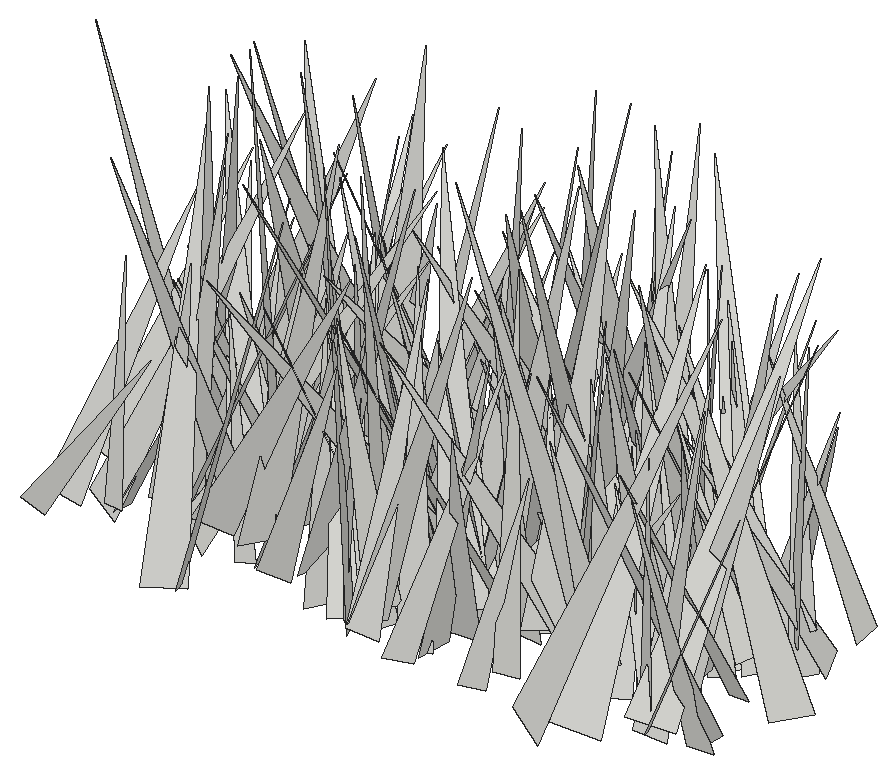
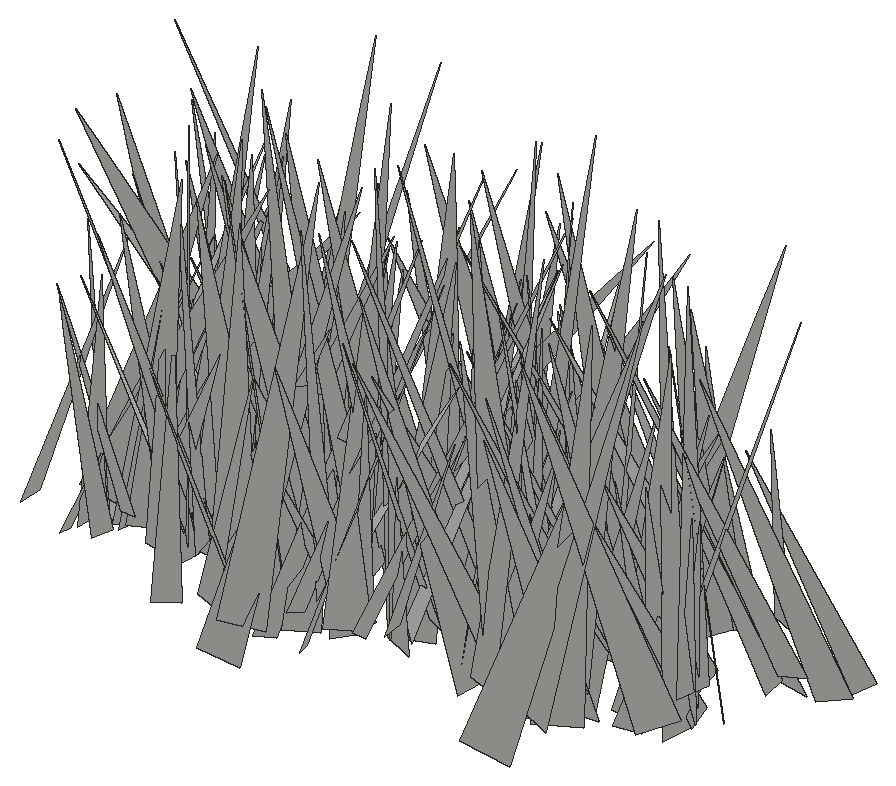
# SketchUp Ruby script. Lengths in inches.
U = 1.inch
M = Sketchup.active_model
def pt(a) = Geom::Point3d.new(a.map { |v| v * U })
def face(e, loops, mat)
  f = e.add_face(loops[0].map { |a| pt(a) })
  loops[1..].each { |l| e.add_face(l.map { |a| pt(a) }).erase! }
  f.material = f.back_material = mat if mat
  f
end
# faces: each face lists its corners as indices into pts; further lists are holes
def faces(e, pts, list, mat = nil) = list.each { |f| face(e, (f[0].is_a?(Array) ? f : [f]).map { |l| l.map { |i| pts[i] } }, mat) }
# xy, xz, yz: faces in a plane at the given z, y or x. An outline is a flat list of corners, or four numbers for a rectangle; further outlines are holes
def ring(l) = l.size == 4 ? [[l[0], l[1]], [l[2], l[1]], [l[2], l[3]], [l[0], l[3]]] : l.each_slice(2).to_a
def flat(e, list, mat, &to3) = list.each { |f| face(e, (f[0].is_a?(Array) ? f : [f]).map { |l| ring(l).map { |u, v| to3.(u, v) } }, mat) }
def xy(e, z, list, mat = nil) = flat(e, list, mat) { |x, y| [x, y, z] }
def xz(e, y, list, mat = nil) = flat(e, list, mat) { |x, z| [x, y, z] }
def yz(e, x, list, mat = nil) = flat(e, list, mat) { |y, z| [x, y, z] }
def lines(e, pts, list) = list.each { |a, b| e.add_line(pt(pts[a]), pt(pts[b])) }
# prism: a flat outline (further loops are holes) pulled along v
def prism(e, loops, v, mat = nil)
  f = face(e, loops, mat); d = Geom::Vector3d.new(v.map { |x| x * U })
  f.pushpull(f.normal.samedirection?(d) ? d.length : -d.length)
end
def box(e, o, s, mat = nil) = prism(e, [[o, [o[0] + s[0], o[1], o[2]], [o[0] + s[0], o[1] + s[1], o[2]], [o[0], o[1] + s[1], o[2]]]], [0, 0, s[2]], mat)
def at(x, y, z, deg = 0) = Geom::Transformation.translation(pt([x, y, z])) * Geom::Transformation.rotation(ORIGIN, Z_AXIS, deg.degrees)
def axes(o, x, y, z) = Geom::Transformation.new([*x, 0, *y, 0, *z, 0, *pt(o).to_a, 1])
def part(name) = M.definitions.add(name)
# library, detail: a bought-in or finely detailed component or shape, given as its bounding box
def library(name, o, s) = part(name).tap { |d| box(d.entities, o, s) }
def detail(e, o, s) = box(e.add_group.entities, o, s)
def put(e, d, t, mat = nil) = e.add_instance(d, t).tap { |i| i.material = mat if mat }
def group(e, t, mat = nil) = e.add_group.tap { |g| g.transformation = t; g.material = mat if mat }.entities
root = M.entities
c1 = part("fur_instance\#9")
p = [[0.8125,0,1.79],[0.67,-0.02,1.48],[0,-0.11,0],[0,0.11,0]]
faces(c1.entities,p,[[0,1,2,3]])
put(root,c1,axes([124.03,185.02,-27.1],[2.18387,-4.44969,1.85832],[-4.59717,-2.53702,-0.67228],[-1.45572,1.33648,4.91091]))
put(root,c1,axes([135.94,185.62,-28.22],[-0.19346,-4.85951,0.89963],[-4.92735,0.1202,-0.41034],[-0.38132,0.91231,4.84602]))
put(root,c1,axes([126.52,182.625,-27.1],[-3.94538,2.89092,1.6801],[2.22143,4.20848,-2.02488],[2.49909,0.82308,4.45234]))
put(root,c1,axes([128.07,184.31,-28.22],[-1.839,3.01934,1.93742],[3.07994,2.44517,-0.88715],[1.83955,-1.07548,3.42218]))
put(root,c1,axes([124.66,183.24,-27.1],[0.1573,5.82785,1.1486],[5.93788,-0.12389,-0.18455],[0.15705,-1.15268,5.82705]))
put(root,c1,axes([124.28,183.96,-27.1],[6.01682,-1.89651,1.60783],[-2.22,-5.99358,1.23799],[-1.11958,1.69241,6.18597]))
put(root,c1,axes([110.55,184.77,-28.22],[1.93678,-3.59499,0.72466],[-3.24209,-1.29543,2.2385],[1.71404,1.61186,3.41529]))
put(root,c1,axes([130.84,183.45,-28.22],[3.76818,7.24013,0.96766],[7.17608,-3.46602,-2.01138],[1.36373,-1.76699,7.91031]))
put(root,c1,axes([125.85,186.65,-28.22],[1.58205,-4.94043,0.08132],[-4.90313,-1.55912,0.66773],[0.6114,0.28046,5.1444]))
put(root,c1,axes([134.61,184.6,-27.1],[2.05844,3.54151,1.67651],[3.74882,-2.33096,0.32115],[-1.13989,-1.27062,4.08367]))
put(root,c1,axes([131.76,186.18,-27.1],[3.25434,-3.10316,1.28908],[-2.93626,-3.49873,-1.00964],[-1.63392,0.10675,4.38189]))
put(root,c1,axes([116.9,185.6,-27.1],[3.69144,-5.31541,0.62902],[-5.0613,-3.21782,2.51095],[1.74141,1.9152,5.96452]))
put(root,c1,axes([125.67,185.44,-28.22],[5.74343,-0.59024,1.12729],[-0.57342,-5.85294,-0.14303],[-1.13593,-0.02976,5.77191]))
put(root,c1,axes([128.98,187.66,-27.1],[-6.06549,-1.51995,0.44377],[-1.27134,5.72216,2.22212],[0.94386,-2.06007,5.84487]))
put(root,c1,axes([119.04,185.95,-28.22],[2.31038,-4.41979,0.71264],[-4.3801,-2.06578,1.38834],[0.92579,1.25629,4.79008]))
put(root,c1,axes([137.13,184.91,-27.1],[-3.79929,-4.93063,0.76728],[-4.2284,2.66909,-3.78564],[-2.64961,2.81057,4.94112]))
put(root,c1,axes([134.55,185.37,-27.1],[2.41252,4.65389,1.89869],[5.02303,-2.30836,-0.72433],[-0.1815,-2.02404,5.19175]))
put(root,c1,axes([113.76,184.69,-27.1],[0.89714,3.83975,1.01573],[3.88067,-1.06922,0.61438],[-0.84607,-0.83267,3.89501]))
put(root,c1,axes([114.77,185.92,-27.1],[1.60896,-4.17155,1.4473],[-4.41412,-1.4813,0.63763],[0.1098,1.57772,4.42538]))
put(root,c1,axes([117.03,187.42,-28.22],[-0.75565,-7.24529,1.23648],[-7.25287,0.53359,-1.30585],[-1.19119,1.34729,7.16659]))
put(root,c1,axes([116.86,183.29,-28.22],[-6.13848,3.83375,0.83292],[3.60337,6.1212,-1.61832],[1.55148,0.95163,7.05405]))
put(root,c1,axes([129.64,184.01,-27.1],[1.15539,6.15443,1.22459],[6.01284,-1.44203,1.57415],[-1.79512,-0.86897,6.06086]))
put(root,c1,axes([123.45,185.78,-27.1],[2.89079,5.81329,3.19782],[6.3896,-3.37876,0.3661],[-1.787,-2.67707,6.48205]))
put(root,c1,axes([122.83,184.93,-28.22],[-6.29577,-3.22015,2.48262],[-3.79064,6.30377,-1.43636],[1.47099,2.46225,6.92409]))
put(root,c1,axes([136.08,187.33,-27.1],[-1.33885,-4.31341,0.19295],[-4.24788,1.27969,-0.86785],[-0.77346,0.43835,4.43226]))
put(root,c1,axes([117.17,183.69,-28.22],[5.32876,3.34285,1.26399],[2.90072,-5.37113,1.97605],[-2.08763,1.0697,5.97207]))
put(root,c1,axes([125.22,185.08,-28.22],[-0.65155,5.99766,1.58433],[6.18323,0.49957,0.65163],[-0.49968,-1.63861,5.99765]))
put(root,c1,axes([122.03,185.44,-28.22],[3.4021,4.35261,1.87369],[4.47593,-3.70904,0.48912],[-1.55627,-1.15238,5.50275]))
put(root,c1,axes([120.39,189.36,-28.22],[-3.43446,-5.67079,0.15135],[-5.3482,3.29577,2.1239],[1.89143,-0.97791,6.28032]))
put(root,c1,axes([121.22,185.38,-28.22],[-4.59387,1.36569,1.34916],[1.20913,4.77619,-0.71765],[1.49109,0.33451,4.73854]))
put(root,c1,axes([130.73,187,-27.1],[-7.92829,-1.68885,1.19775],[-1.65667,8.01779,0.33921],[1.24187,-0.08605,8.09907]))
put(root,c1,axes([127.43,186.875,-27.1],[-4.42248,-6.55022,0.11235],[-5.68971,3.77318,-3.9833],[-3.24733,2.30957,6.8262]))
put(root,c1,axes([120.95,185.48,-27.1],[6.83211,0.09479,1.62922],[-0.11306,-6.96812,0.87954],[-1.62805,0.88169,6.77592]))
put(root,c1,axes([118.62,185.8,-27.1],[6.64236,-2.17739,2.19825],[-2.53423,-6.81539,0.90685],[-1.77512,1.5823,6.93106]))
put(root,c1,axes([134.13,185.76,-28.22],[-3.36159,2.04077,0.19725],[2.04893,3.35754,0.1809],[0.07444,-0.25709,3.9284]))
put(root,c1,axes([123.34,189.74,-28.22],[2.28844,-6.77562,0.58153],[-5.77223,-2.2597,-3.61376],[-3.59563,-0.68473,6.17144]))
put(root,c1,axes([122.98,188.57,-27.1],[-2.64137,-6.46023,1.04071],[-6.35863,2.79897,1.23619],[1.54452,0.47506,6.86901]))
put(root,c1,axes([124.71,186.93,-27.1],[-2.99975,-3.60869,1.08185],[-3.74003,3.01886,-0.30041],[0.45307,1.02732,4.68304]))
put(root,c1,axes([125.92,187.65,-27.1],[-2.72161,-4.19987,1.18368],[-4.18397,2.90781,0.69726],[1.23872,0.59401,4.95579]))
put(root,c1,axes([131.29,185.13,-28.22],[-5.36603,-1.88935,2.74168],[-2.67241,5.54565,-1.40882],[1.98613,2.35731,5.51173]))
put(root,c1,axes([124.97,188.17,-27.1],[-3.4454,-3.89131,0.03074],[-3.88746,3.44363,0.20759],[0.17579,-0.11462,5.19326]))
put(root,c1,axes([132.21,184.17,-28.22],[-1.86477,7.56726,1.18834],[7.49142,2.05683,-1.34204],[1.5982,-0.81177,7.67722]))
put(root,c1,axes([132.52,188.1,-28.22],[2.01145,-6.31603,1.30369],[-6.40118,-2.12156,-0.40211],[-0.78536,1.11557,6.61638]))
put(root,c1,axes([115.02,186.57,-27.1],[5.24676,-2.59436,1.90695],[-2.83441,-5.4512,0.38233],[-1.5275,1.20389,5.84064]))
put(root,c1,axes([134.21,185.32,-28.22],[-0.07417,5.83715,1.21265],[5.95855,0.11247,-0.17697],[0.19614,-1.2097,5.83493]))
put(root,c1,axes([122.29,185.27,-28.22],[-3.8761,2.85036,0.12124],[2.83481,3.87102,-0.37744],[0.32105,0.23257,4.79648]))
put(root,c1,axes([129.32,186.71,-28.22],[1.13497,4.33314,1.68645],[4.04549,-0.06445,-2.557],[2.29221,-2.03177,3.67778]))
put(root,c1,axes([118.98,187.38,-27.1],[3.98619,-2.41358,0.43201],[-2.42835,-4.00018,0.05811],[-0.33929,0.27366,4.65958]))
put(root,c1,axes([123.68,185.76,-28.22],[-4.83845,-0.36416,0.05457],[-0.36621,4.6838,-1.21411],[-0.03844,1.21473,4.69778]))
put(root,c1,axes([133.05,186.24,-27.1],[-3.3024,-1.44134,1.34219],[-1.74105,3.36144,-0.674],[0.92071,1.18661,3.53964]))
put(root,c1,axes([117.83,186.05,-28.22],[0.1057,3.9764,0.92499],[3.9126,-0.36287,1.11284],[-1.16573,-0.85739,3.81897]))
put(root,c1,axes([110.84,185.86,-28.22],[-0.64371,5.67181,1.6895],[5.48083,1.21245,-1.9821],[2.23257,-1.34117,5.35305]))
put(root,c1,axes([133.94,186.61,-28.22],[-2.23276,3.13779,0.67741],[3.20125,2.1153,0.75324],[-0.23799,-0.9847,3.77672]))
put(root,c1,axes([133.21,188.96,-28.22],[5.7747,-1.11479,0.95698],[-0.77258,-5.60537,-1.86777],[-1.24967,-1.68603,5.57685]))
put(root,c1,axes([112.75,186.39,-28.22],[4.1398,0.29454,0.02134],[0.28882,-4.10074,0.57065],[-0.06159,0.56772,4.11084]))
put(root,c1,axes([121.53,187.34,-27.1],[-4.43723,-6.45792,2.6794],[-6.95056,4.4181,-0.86196],[0.75734,2.71083,7.78786]))
put(root,c1,axes([134.17,186.74,-27.1],[3.16186,-4.77933,2.12939],[-5.21892,-2.70344,1.68164],[0.37303,2.68757,5.47827]))
put(root,c1,axes([126.05,186.4,-27.1],[-4.29093,5.93832,1.73067],[6.14946,4.32229,0.41585],[0.66564,-1.65078,7.31456]))
put(root,c1,axes([135.22,183.87,-27.1],[5.40862,3.75774,0.29196],[3.28966,-4.95573,2.84217],[-1.83956,2.18614,5.94103]))
put(root,c1,axes([130.49,187.9,-27.1],[3.95695,-1.9726,1.7752],[-1.97238,-4.31833,-0.40205],[-1.77544,0.40099,4.40306]))
put(root,c1,axes([118.12,186.35,-28.22],[4.19181,1.99584,0.5753],[1.88629,-4.2003,0.82769],[-0.86965,0.50967,4.56832]))
put(root,c1,axes([126.03,187.22,-27.1],[3.90442,0.1948,1.09665],[0.0575,-4.02752,0.51071],[-1.11233,0.47558,3.87577]))
put(root,c1,axes([127.55,187.76,-28.22],[-1.40726,-4.75955,2.034],[-5.17479,1.24906,-0.65748],[-0.10975,2.13481,4.91949]))
put(root,c1,axes([115.68,185.71,-27.1],[5.65943,2.62486,0.30549],[2.50558,-5.55953,1.3513],[-0.8398,1.10185,6.0904]))
put(root,c1,axes([117.69,188.73,-27.1],[-0.92246,-4.02488,0.49642],[-3.83236,0.69867,-1.45667],[-1.32631,0.78053,3.86377]))
put(root,c1,axes([132.05,188.26,-27.1],[4.08918,-3.36848,1.98263],[-3.52303,-4.41912,-0.24183],[-1.69286,1.05996,5.29241]))
put(root,c1,axes([115.49,186.4,-28.22],[4.07618,6.66518,0.05677],[6.29765,-3.82934,-2.59208],[2.18344,-1.39809,7.37028]))
put(root,c1,axes([120.55,189.5625,-27.1],[2.722,-4.21365,0.18087],[-4.20663,-2.72794,-0.24377],[-0.30292,0.01939,5.01046]))
put(root,c1,axes([132.64,188.15,-27.1],[4.18709,2.7222,0.51054],[2.74144,-3.94162,-1.4666],[0.39441,-1.502,4.77401]))
put(root,c1,axes([135.03,184.31,-27.1],[-5.0261,5.87636,0.71878],[5.2638,4.86732,-2.98524],[2.70938,1.44485,7.13314]))
put(root,c1,axes([121.66,188.67,-28.22],[3.72524,-2.31212,0.81738],[-2.32656,-3.80205,-0.15146],[-0.77532,0.29988,4.38182]))
put(root,c1,axes([126.26,187.01,-27.1],[-4.785,3.6619,0.62252],[3.69492,4.79647,0.18627],[0.38032,-0.52686,6.02254]))
put(root,c1,axes([122.25,187.16,-28.22],[-2.95191,2.4359,0.97471],[2.3622,3.10602,-0.60836],[1.1418,-0.12828,3.77853]))
put(root,c1,axes([112.2,186.13,-28.22],[3.27574,7.01328,0.4286],[6.91428,-3.13335,-1.57325],[1.25002,-1.04703,7.57902]))
put(root,c1,axes([128.17,190.72,-27.1],[-1.4202,-8.16889,0.91065],[-8.13373,1.52988,1.03868],[1.18423,0.71114,8.22611]))
put(root,c1,axes([118.68,186.77,-27.1],[-6.74078,-2.87477,2.26806],[-3.46071,6.55422,-1.97791],[1.19661,2.76122,7.05622]))
put(root,c1,axes([135.44,190.52,-28.22],[-4.47092,-4.93614,0.16266],[-4.90041,4.46105,0.68268],[0.61475,-0.33851,6.62484]))
put(root,c1,axes([125.06,188.28,-27.1],[-5.1041,-1.8904,0.52095],[-1.9461,5.06157,-0.70004],[0.24022,0.83889,5.39772]))
put(root,c1,axes([131.35,189.27,-27.1],[3.43553,-2.13589,0.95207],[-2.02418,-3.56342,-0.68999],[-1.17096,-0.10667,3.98608]))
put(root,c1,axes([121.74,186.18,-27.1],[-4.67511,2.29396,0.21165],[2.12082,4.47274,-1.63107],[0.89953,1.37696,4.94555]))
put(root,c1,axes([116.57,188.1875,-28.22],[-2.17172,3.54056,2.13295],[3.72846,2.71807,-0.7156],[1.78427,-1.37037,4.09143]))
put(root,c1,axes([128.85,186.93,-27.1],[5.55139,-3.03279,3.66915],[-4.09539,-5.91606,1.30628],[-2.42657,3.04644,6.18946]))
put(root,c1,axes([132.2,190.83,-28.22],[7.53052,-1.13144,2.64431],[-0.30654,-7.68469,-2.41514],[-2.85982,-2.15562,7.22191]))
put(root,c1,axes([115.49,188.07,-28.22],[-7.70081,-2.50661,0.76749],[-2.60656,7.57519,-1.4131],[0.27927,1.58364,7.97425]))
put(root,c1,axes([121.11,187.35,-28.22],[3.60121,-2.60608,3.3834],[-3.59297,-4.24118,0.55747],[-2.30861,2.53545,4.41017]))
put(root,c1,axes([127.66,189.49,-27.1],[-3.40896,-3.60182,1.17644],[-3.63778,3.55381,0.3393],[1.06005,0.61272,4.94762]))
put(root,c1,axes([133.87,188.17,-28.22],[-3.20539,-1.99252,1.2784],[-2.28309,3.17085,-0.78241],[0.62603,1.36182,3.69222]))
put(root,c1,axes([111.49,187.08,-27.1],[0.65579,5.75921,0.77226],[5.58682,-0.41126,-1.67728],[1.5976,-0.92592,5.54845]))
put(root,c1,axes([136.88,188.89,-28.22],[-3.75455,5.21199,1.89568],[5.51913,3.28609,1.89629],[-0.5456,-2.62523,6.13723]))
put(root,c1,axes([122.79,186.89,-27.1],[3.66563,6.83822,1.35122],[6.90712,-3.76874,0.33492],[-0.93742,-1.02919,7.75151]))
put(root,c1,axes([125.94,187.72,-28.22],[6.87844,-2.02965,2.77665],[-2.6588,-7.07628,1.41394],[-2.18175,2.22463,7.03088]))
put(root,c1,axes([123.39,193.34,-27.1],[-6.54697,-3.05595,0.68846],[-2.14459,5.53525,4.1758],[2.28332,-3.56338,5.89613]))
put(root,c1,axes([112.99,188.63,-28.22],[4.60486,4.04407,1.88978],[4.30358,-4.74303,-0.33665],[-1.18533,-1.50984,6.1193]))
put(root,c1,axes([116.68,188.83,-27.1],[2.49544,-4.2024,1.5625],[-4.46283,-2.15679,1.32672],[0.42981,2.0042,4.70396]))
put(root,c1,axes([115.18,190.61,-28.22],[-0.2394,-4.99537,0.47277],[-5.01072,0.21306,-0.28607],[-0.26442,0.48521,4.99291]))
put(root,c1,axes([131.63,186.36,-28.22],[-5.97227,4.9002,0.90124],[4.6479,5.98621,-1.7477],[1.79477,0.80344,7.52499]))
put(root,c1,axes([113.26,190.49,-28.22],[7.9282,0.66664,2.15118],[1.11346,-8.00329,-1.62351],[-1.9576,-1.85234,7.78877]))
put(root,c1,axes([119.15,190.22,-27.1],[4.7247,0.27251,1.48983],[0.66278,-4.76043,-1.23114],[-1.36183,-1.37139,4.56961]))
put(root,c1,axes([113.26,189.75,-27.1],[6.40054,-0.55178,2.21578],[-0.37829,-6.75939,-0.5905],[-2.25189,-0.43282,6.39709]))
put(root,c1,axes([116.64,191.03,-28.22],[3.23703,-3.40023,0.62778],[-3.13183,-3.24768,-1.44163],[-1.46538,-0.57015,4.46784]))
put(root,c1,axes([116.55,192.03,-27.1],[2.6634,-7.09113,0.13913],[-7.08626,-2.66678,-0.26525],[-0.29724,0.03689,7.57017]))
put(root,c1,axes([114.62,191.23,-28.22],[3.29812,-3.00828,0.87507],[-2.53709,-3.30998,-1.81667],[-1.83812,-0.82908,4.07763]))
put(root,c1,axes([122.99,190.91,-28.22],[1.53045,-4.60076,0.23907],[-4.60681,-1.52625,0.11946],[0.03806,0.26453,4.84716]))
put(root,c1,axes([116.23,188.34,-28.22],[-3.46559,5.8146,1.30946],[5.95968,3.40104,0.67057],[0.08042,-1.46897,6.73574]))
put(root,c1,axes([127.91,188.48,-28.22],[-1.47936,3.73163,0.54523],[3.76451,1.42617,0.45319],[-0.22551,-0.67216,3.98851]))
put(root,c1,axes([132.38,189.06,-27.1],[-1.64307,3.38565,0.94063],[3.51296,1.55882,0.52563],[-0.08077,-1.0745,3.72639]))
put(root,c1,axes([134.79,189.34,-27.1],[-3.98782,0.86871,0.11292],[0.87287,3.98492,0.16912],[0.07423,-0.18933,4.07783]))
put(root,c1,axes([130.04,190,-28.22],[-3.06281,-3.15709,1.43812],[-3.29391,3.24851,0.11628],[1.08883,0.94666,4.3971]))
put(root,c1,axes([129.55,192.49,-28.22],[-0.91329,-6.82842,0.06821],[-6.63421,0.90353,1.6239],[1.61843,-0.14959,6.69511]))
put(root,c1,axes([114.55,187.45,-28.22],[4.59265,0.40937,1.72839],[-0.43371,-4.3881,2.19176],[-1.72245,2.19644,4.05662]))
put(root,c1,axes([127.6875,190.375,-28.22],[7.89082,-0.9052,1.78608],[-0.78265,-8.07818,-0.63641],[-1.84308,-0.44515,7.91703]))
put(root,c1,axes([125.3,191.5625,-27.1],[4.0127,-3.86264,0.72099],[-3.71726,-4.06564,-1.09277],[-1.27351,-0.30356,5.46147]))
put(root,c1,axes([115.47,189.39,-28.22],[3.2036,5.15972,0.63397],[4.7617,-2.61371,-2.78969],[2.08586,-1.95793,5.39475]))
put(root,c1,axes([119.8,190.82,-27.1],[-1.12963,-3.6746,0.26296],[-3.62855,1.06225,-0.74377],[-0.63679,0.46567,3.77168]))
put(root,c1,axes([133.63,189.54,-28.22],[-1.38179,3.78074,1.32931],[4.00762,1.30133,0.46468],[-0.00636,-1.40818,3.99842]))
put(root,c1,axes([113.95,189.09,-28.22],[0.5553,3.90242,1.15183],[3.90207,-0.84018,0.96535],[-1.15302,-0.96393,3.8217]))
put(root,c1,axes([125.83,193.41,-27.1],[-6.83742,-2.67371,1.15288],[-1.91772,6.34944,3.35188],[2.19094,-2.7864,6.53176]))
put(root,c1,axes([119.61,190.12,-28.22],[1.20072,-3.47995,0.99765],[-3.52529,-0.88496,1.15597],[0.82322,1.28603,3.49507]))
put(root,c1,axes([113.68,189.53,-28.22],[0.50374,3.60666,1.32904],[3.78488,-0.69911,0.46265],[-0.67011,-1.23747,3.61216]))
put(root,c1,axes([130.6,190.43,-28.22],[-6.43604,2.78332,0.65453],[2.85741,6.20344,1.71766],[-0.1023,-1.83529,6.79846]))
put(root,c1,axes([126.2,192.67,-28.22],[6.011,-2.52803,0.45147],[-2.2406,-5.7244,-2.22212],[-1.25478,-1.8887,6.13068]))
put(root,c1,axes([123.98,193.33,-27.1],[7.80685,-2.34529,0.78759],[-1.91376,-7.37702,-2.99744],[-1.56786,-2.67335,7.58041]))
put(root,c1,axes([135.75,192.24,-28.22],[-4.91943,-1.92287,0.32626],[-1.70701,4.67316,1.80343],[0.9434,-1.57124,4.96446]))
put(root,c1,axes([115.52,189.125,-27.1],[0.0321,3.78164,0.61426],[3.82721,-0.05969,0.16749],[-0.17489,-0.6122,3.77806]))
put(root,c1,axes([127.8,192.59,-28.22],[4.34994,-4.04005,0.73934],[-3.73736,-4.34022,-1.72779],[-1.70317,-0.79441,5.67968]))
put(root,c1,axes([122.83,187.36,-28.22],[5.49101,0.89671,2.25711],[-0.37206,-5.20349,2.97239],[-2.40004,2.85822,4.70322]))
put(root,c1,axes([129.6,188.09,-27.1],[5.08694,2.79276,1.06084],[2.31416,-5.00849,2.08845],[-1.88933,1.38471,5.41433]))
put(root,c1,axes([122.38,192.19,-27.1],[-4.64993,-4.92524,0.42817],[-4.93518,4.6591,-0.00251],[0.29211,0.31306,6.77347]))
put(root,c1,axes([135.03,191.4,-27.1],[-3.6368,4.97548,2.15784],[5.29036,2.68314,2.72961],[-1.1932,-3.26854,5.52548]))
put(root,c1,axes([126.01,188.21,-28.22],[-6.72177,-1.11045,3.37602],[-2.29516,6.87097,-2.30972],[2.71346,3.06096,6.4094]))
put(root,c1,axes([126.86,193.61,-28.22],[-6.3203,-1.31951,1.76492],[-0.3807,5.93404,3.07318],[2.17051,-2.80147,5.67828]))
put(root,c1,axes([133.67,190.5625,-27.1],[-3.19624,2.75407,0.40141],[2.73336,2.9911,1.24258],[-0.52417,-1.19599,4.03198]))
put(root,c1,axes([115.23,188.875,-27.1],[-0.56854,4.75375,0.07359],[4.64609,0.5398,1.02436],[-1.0087,-0.19303,4.67676]))
put(root,c1,axes([113.36,189.3125,-28.22],[4.45385,0.90104,0.34779],[0.77968,-4.32278,1.21461],[-0.57002,1.12752,4.37874]))
put(root,c1,axes([131.26,191.93,-27.1],[-4.22534,-4.50008,2.6097],[-4.33201,4.90527,1.44456],[2.88009,0.77613,6.00146]))
put(root,c1,axes([126.45,190.625,-27.1],[6.91635,-1.96319,0.7746],[-2.05636,-6.86586,0.95992],[-0.47486,1.1384,7.12521]))
put(root,c1,axes([119.38,190.28,-28.22],[3.41975,6.53108,1.33927],[6.45057,-2.86091,-2.51965],[1.68487,-2.30293,6.92828]))
put(root,c1,axes([125.45,193.5,-28.22],[-5.24067,-3.21189,0.67738],[-2.84495,5.08085,2.08111],[1.63749,-1.45206,5.78359]))
put(root,c1,axes([125.375,190.21,-27.1],[7.84011,2.17766,1.89393],[2.14429,-8.06482,0.39652],[-1.93163,-0.114,8.12726]))
put(root,c1,axes([123.3,191.57,-28.22],[-3.32783,-6.52848,3.29816],[-6.89122,4.01297,0.99019],[2.45153,2.41834,7.26051]))
put(root,c1,axes([120.53,192.16,-28.22],[-3.91635,-3.27614,1.36892],[-3.24396,4.13005,0.60351],[1.44353,0.39293,5.07017]))
put(root,c1,axes([126.08,190.91,-27.1],[-4.47703,-2.46915,0.00102],[-2.34184,4.24552,-1.62229],[-0.78262,1.42103,4.84857]))
put(root,c1,axes([117.35,191.13,-27.1],[5.44742,2.57642,1.57153],[2.74581,-5.57692,-0.37485],[-1.25227,-1.0208,6.0143]))
put(root,c1,axes([131.55,190.2,-27.1],[-7.28379,2.71503,1.56111],[2.64145,7.44897,-0.63058],[1.68261,0.05921,7.74773]))
put(root,c1,axes([130.53,192.07,-27.1],[5.81902,2.09502,1.94943],[2.48849,-5.88572,-1.1028],[-1.4131,-1.7377,6.08555]))
put(root,c1,axes([123.53,190.76,-28.22],[4.3952,-2.19196,2.60814],[-2.70598,-4.83259,0.49862],[-2.06997,1.6632,4.88608]))
put(root,c1,axes([125.01,192.125,-28.22],[3.09975,-1.98369,0.33098],[-1.98147,-3.11644,-0.1208],[-0.34401,0.07615,3.67817]))
put(root,c1,axes([121.86,190.73,-27.1],[0.71871,3.7725,0.80138],[3.83913,-0.62217,-0.51422],[0.36739,-0.87844,3.80576]))
put(root,c1,axes([135.17,191.11,-27.1],[2.79154,3.79561,1.789],[3.98615,-3.06992,0.29332],[-1.31064,-1.25251,4.70248]))
put(root,c1,axes([116.65,189.77,-27.1],[1.55452,5.85258,0.28483],[5.77094,-1.47817,-1.12324],[1.01494,-0.55917,5.95042]))
put(root,c1,axes([118.94,191.41,-28.22],[-5.12716,5.45276,3.67809],[5.84452,5.9162,-0.62364],[3.01704,-2.19425,7.45865]))
put(root,c1,axes([124.1,192.24,-27.1],[0.22689,-3.51122,0.97081],[-3.62685,-0.12635,0.39066],[0.3422,0.98893,3.49679]))
put(root,c1,axes([134.36,190.48,-28.22],[-5.52094,1.92393,0.48296],[1.85996,5.5174,-0.71721],[0.68943,0.52184,5.80241]))
put(root,c1,axes([130.54,190.94,-27.1],[-2.56552,5.11443,0.44811],[4.78646,2.20153,2.27666],[-1.85689,-1.39139,5.24939]))
put(root,c1,axes([122.05,191.32,-27.1],[2.7927,4.03544,0.85961],[4.11922,-2.66751,-0.85986],[0.23622,-1.19268,4.83163]))
put(root,c1,axes([118.55,193.4,-27.1],[-2.6676,-6.3456,1.58153],[-6.4273,2.85927,0.63121],[1.20736,1.20081,6.85451]))
put(root,c1,axes([133.08,190.75,-27.1],[-0.96186,4.58475,0.31518],[4.19254,0.74357,1.97843],[-1.88199,-0.68675,4.24628]))
put(root,c1,axes([131.32,189.17,-27.1],[-7.41355,2.38035,1.13819],[1.92535,7.2016,-2.52036],[1.80404,2.09598,7.36713]))
put(root,c1,axes([131.7,191.59,-28.22],[5.84499,-0.86217,1.83487],[-1.09003,-6.05756,0.62599],[-1.70936,0.91471,5.87498]))
put(root,c1,axes([136.68,192.8,-27.1],[-4.93591,-0.64757,0.62999],[-0.58328,4.95621,0.52453],[0.68994,-0.44273,4.95049]))
put(root,c1,axes([117.76,192.99,-28.22],[3.45559,-4.90486,0.92565],[-4.98413,-3.32981,0.96246],[0.2699,1.30779,5.9222]))
put(root,c1,axes([133.66,191.82,-27.1],[1.6531,3.56586,0.9383],[3.65871,-1.45863,-0.90264],[0.45784,-1.21883,3.82535]))
put(root,c1,axes([119.91,192.04,-28.22],[6.4862,-0.82849,0.61771],[-0.87391,-6.49276,0.46816],[-0.55158,0.54452,6.52212]))
put(root,c1,axes([119.42,191.53,-27.1],[-0.23432,4.6061,1.3303],[4.44797,-0.2882,1.78136],[-1.78924,-1.31967,4.25416]))
put(root,c1,axes([125.8,190.93,-28.22],[-0.30009,3.62925,0.24074],[3.53668,0.34756,-0.831],[0.84929,-0.16496,3.54556]))
put(root,c1,axes([117.1,195.09,-28.22],[0.76231,-8.24421,0.75454],[-8.09051,-0.90251,-1.68715],[-1.75496,0.57958,8.10565]))
put(root,c1,axes([128.08,193.54,-27.1],[5.88193,4.68919,0.48239],[4.10623,-4.71789,-4.20698],[2.31519,-3.54559,6.23594]))
put(root,c1,axes([135.55,191.125,-28.22],[-5.20641,1.3754,0.94823],[1.21962,5.25029,-0.91901],[1.14166,0.66356,5.30602]))
put(root,c1,axes([134.05,190.62,-28.22],[-4.81407,6.51041,0.79127],[6.55623,4.75265,0.78417],[-0.16528,-1.10168,8.05889]))
put(root,c1,axes([116.08,191.43,-28.22],[1.48764,5.46016,1.29529],[5.56167,-1.25605,-1.09283],[0.74757,-1.52092,5.55267]))
put(root,c1,axes([131.09,190.74,-28.22],[1.31333,6.20143,0.89],[6.24264,-1.21867,-0.72041],[0.52849,-1.01577,6.2979]))
put(root,c1,axes([116.4375,192.38,-28.22],[-4.39266,5.33205,2.64396],[5.82364,4.52851,0.54275],[1.2274,-2.40386,6.88706]))
put(root,c1,axes([122.81,192.46,-27.1],[-3.89073,-0.42692,0.42553],[-0.44504,3.90915,-0.14719],[0.40654,0.19356,3.91132]))
put(root,c1,axes([131.64,192.9375,-27.1],[-0.96334,-4.21277,1.52504],[-4.43315,1.12201,0.29911],[0.64835,1.41239,4.31115]))
put(root,c1,axes([129.72,191.58,-27.1],[-5.3119,3.70536,1.5571],[3.75007,5.49761,-0.28937],[1.44609,-0.64586,6.4701]))
put(root,c1,axes([127.46,192.02,-27.1],[-4.33935,-4.28478,3.74469],[-5.00881,5.11096,0.04388],[2.70071,2.59437,6.09815]))
put(root,c1,axes([127.16,195.52,-28.22],[-0.22294,-7.81188,0.28991],[-7.80547,0.20653,-0.4373],[-0.42917,0.30182,7.80282]))
put(root,c1,axes([132.02,191.17,-27.1],[3.70568,3.40586,0.49894],[3.35111,-3.73706,0.62078],[-0.78668,0.12425,4.99466]))
put(root,c1,axes([115.99,194.12,-27.1],[-2.53564,-6.45433,1.27855],[-6.57975,2.48748,-0.49186],[0.00081,1.3699,6.91708]))
put(root,c1,axes([133.48,193.27,-27.1],[3.83276,-0.80553,0.30542],[-0.78769,-3.84079,-0.24507],[-0.34886,-0.17786,3.90882]))
put(root,c1,axes([125.04,191.4,-28.22],[-3.03856,4.16793,1.35783],[3.96538,3.31773,-1.3102],[1.86846,-0.26309,4.98878]))
put(root,c1,axes([130.54,193.84,-28.22],[2.48728,-3.44318,0.65298],[-3.47724,-2.52444,-0.0662],[-0.43662,0.49004,4.24707]))
put(root,c1,axes([118.94,191.99,-27.1],[0.50211,5.33526,1.29674],[5.04367,0.06639,-2.22613],[2.16978,-1.38897,4.87457]))
put(root,c1,axes([112.73,192.08,-27.1],[4.48664,-4.30175,1.96808],[-4.72578,-3.95369,2.13158],[0.21294,2.89338,5.83878]))
put(root,c1,axes([126.22,191.45,-27.1],[-6.64988,-1.58039,2.79885],[-2.32051,6.81074,-1.66765],[2.22405,2.38079,6.62853]))
put(root,c1,axes([129.58,193.01,-28.22],[-1.21907,-3.82959,1.50139],[-4.09681,0.98993,-0.80143],[-0.36895,1.66143,3.93822]))
put(root,c1,axes([117.41,190.48,-28.22],[-3.21539,5.33291,0.27404],[5.21793,3.20577,-1.16191],[1.13501,0.36996,6.11789]))
put(root,c1,axes([126.61,195.07,-27.1],[2.5513,-6.67742,1.15565],[-6.68995,-2.67869,-0.70836],[-1.08074,0.81812,7.11304]))
